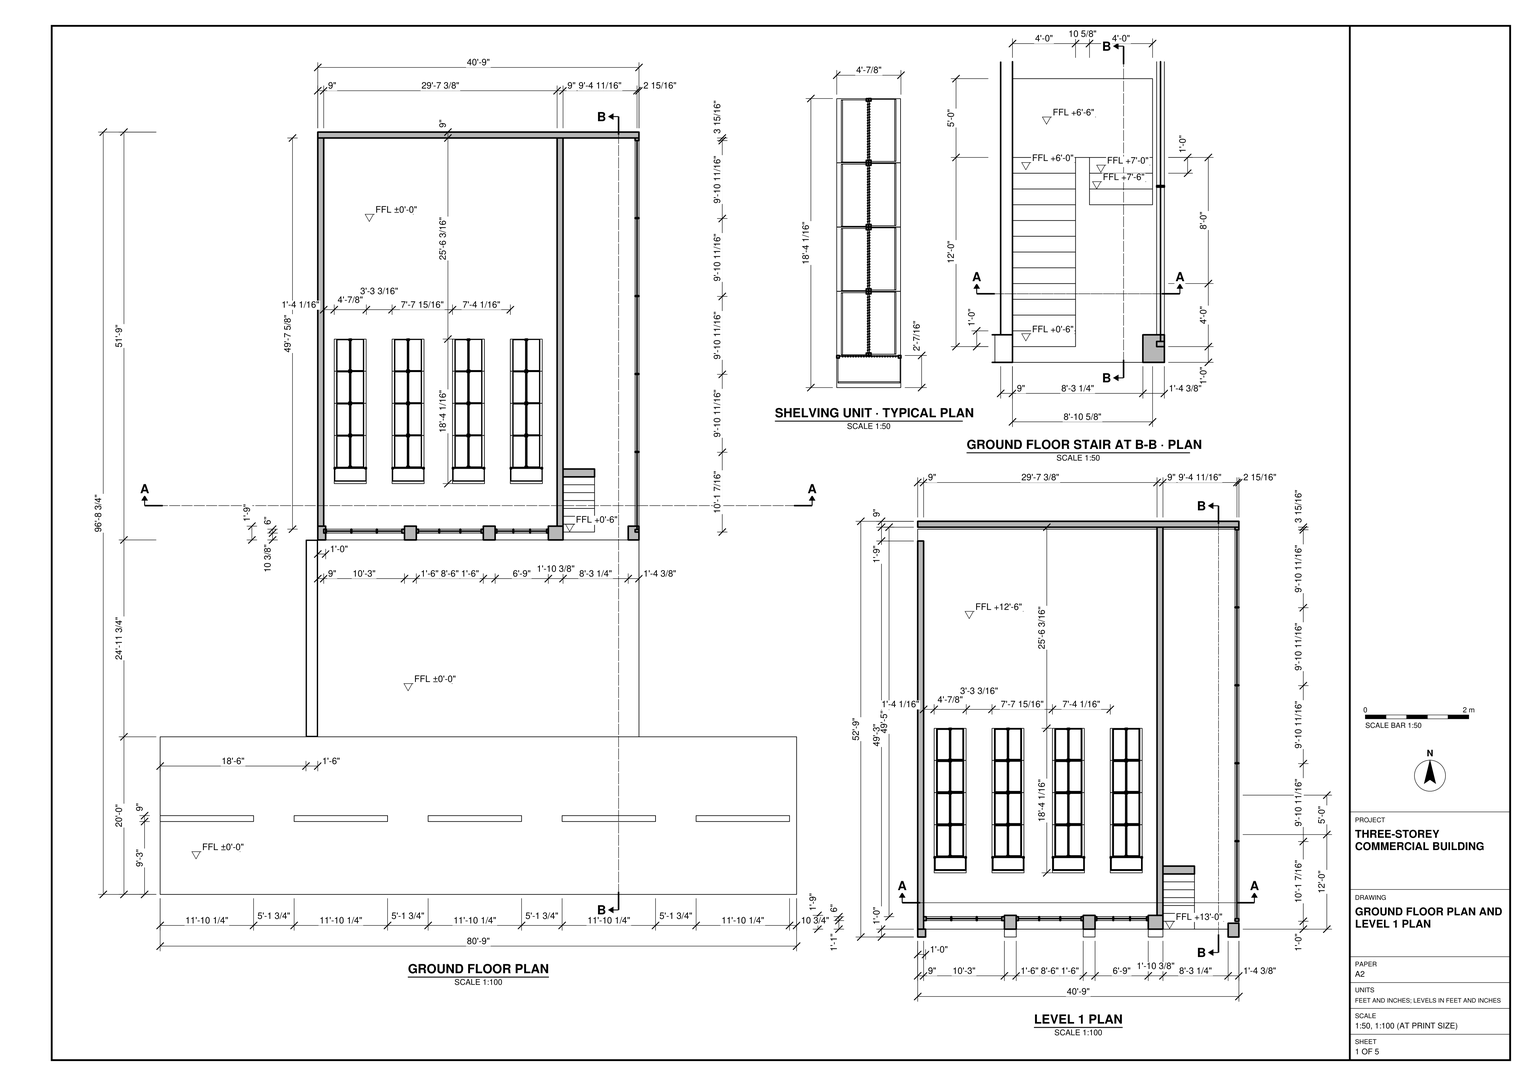
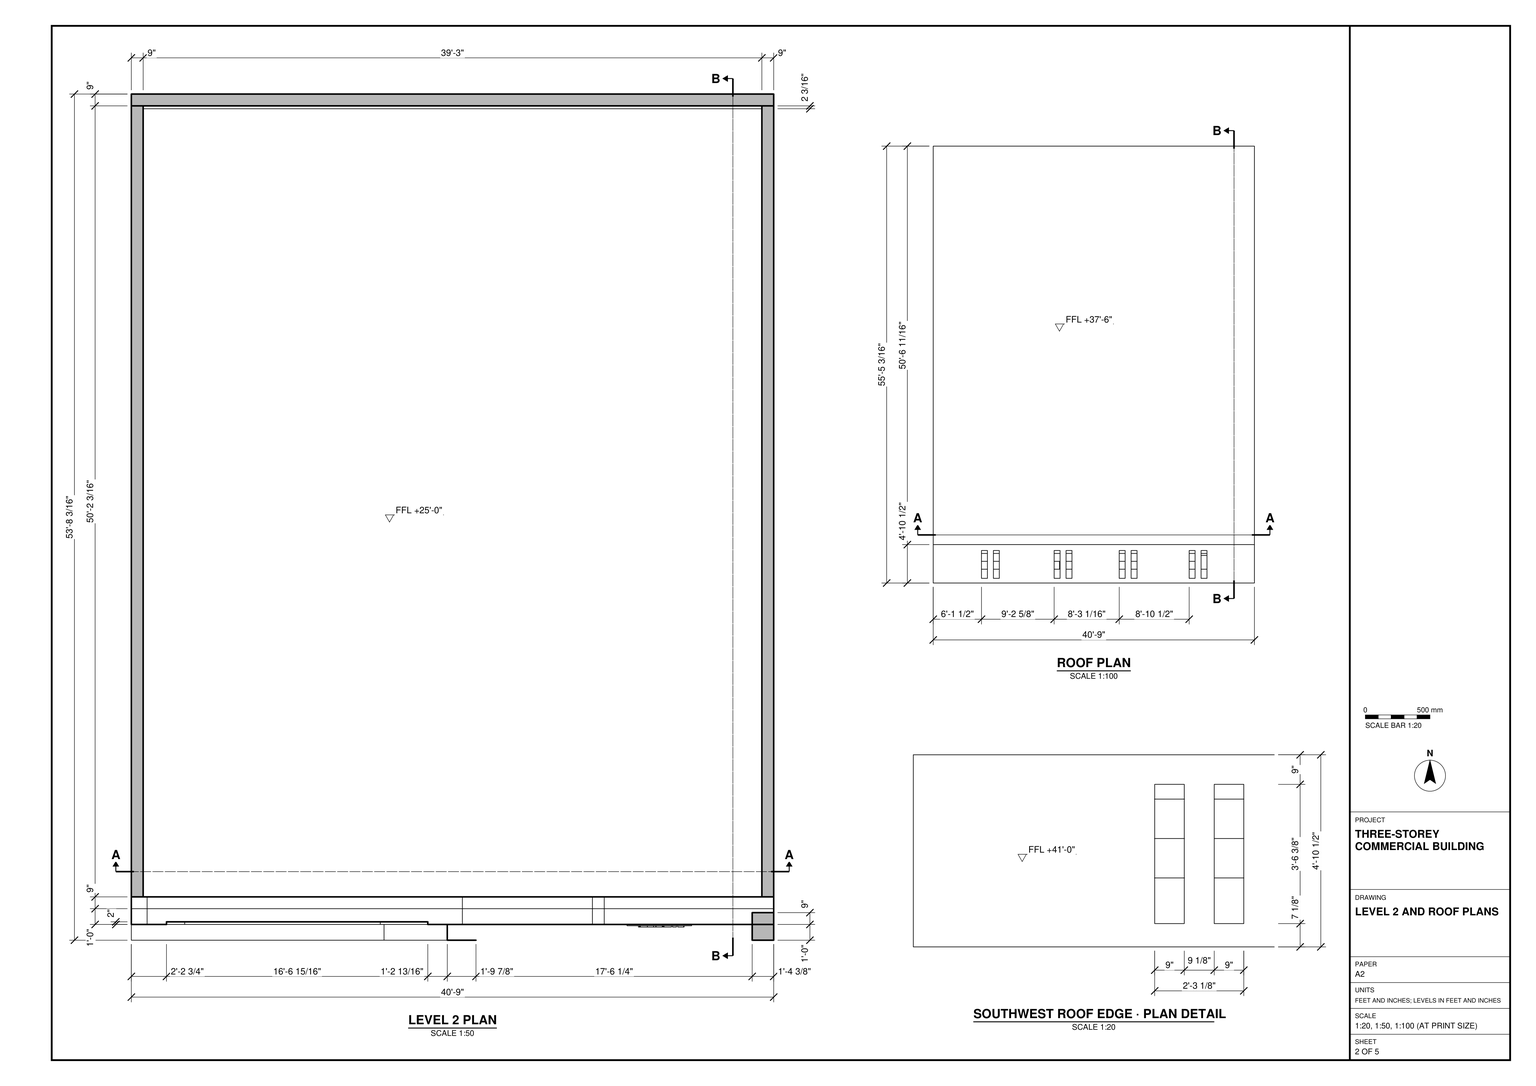
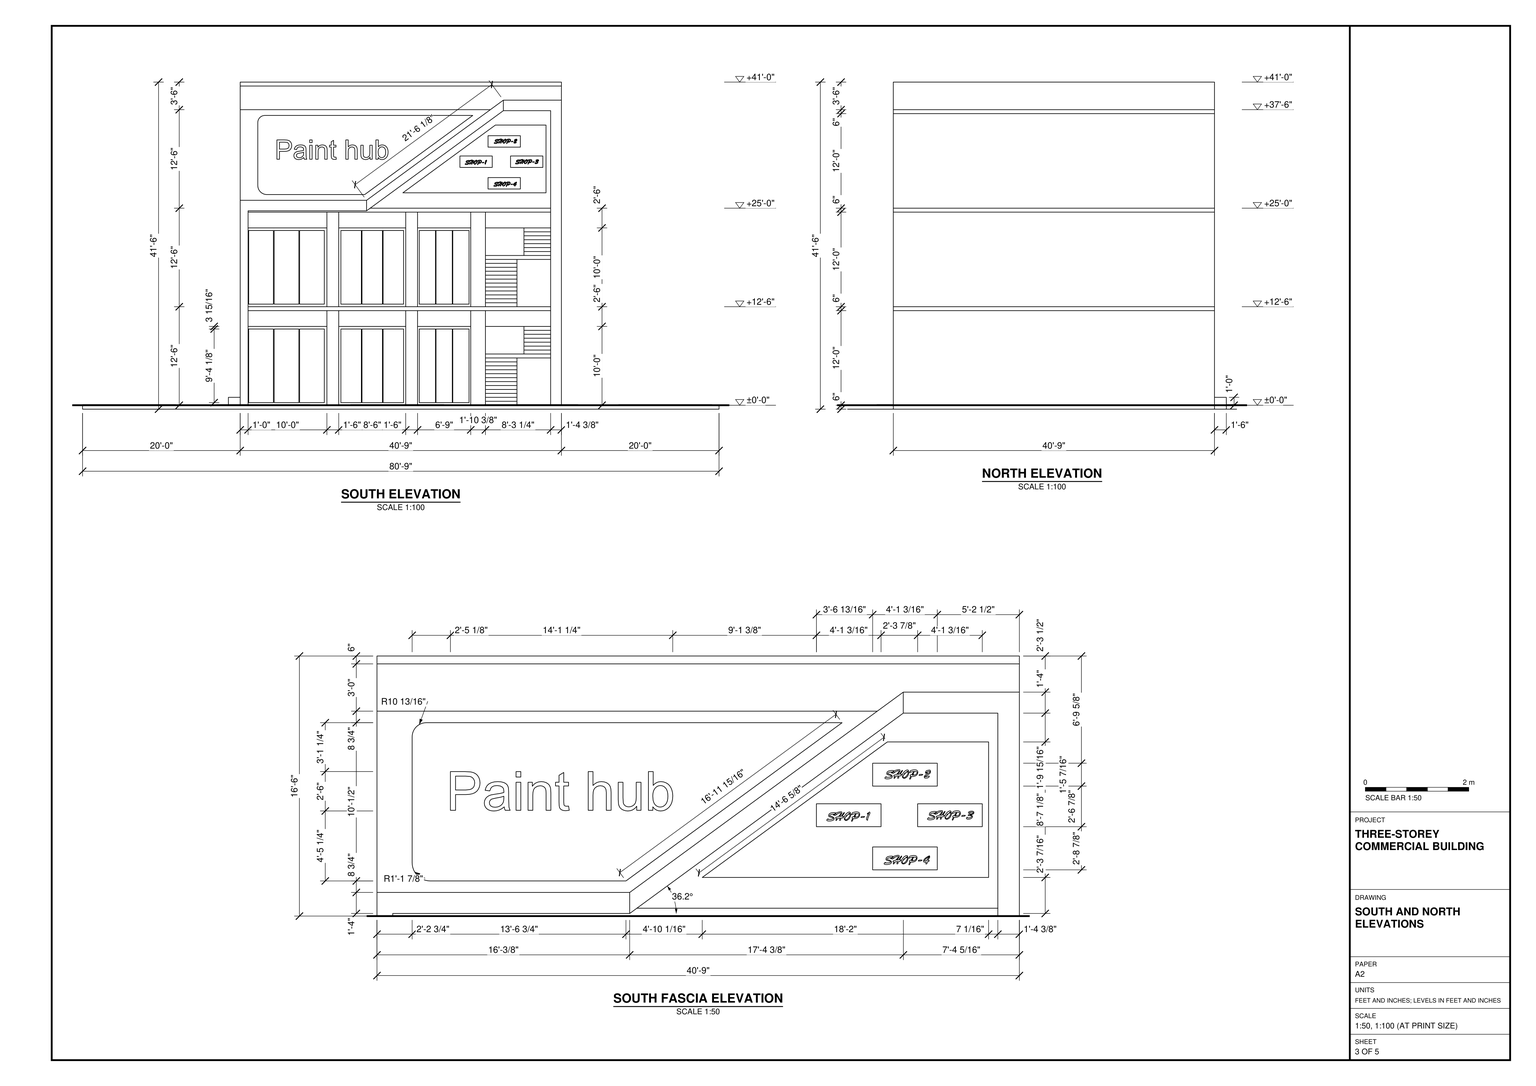
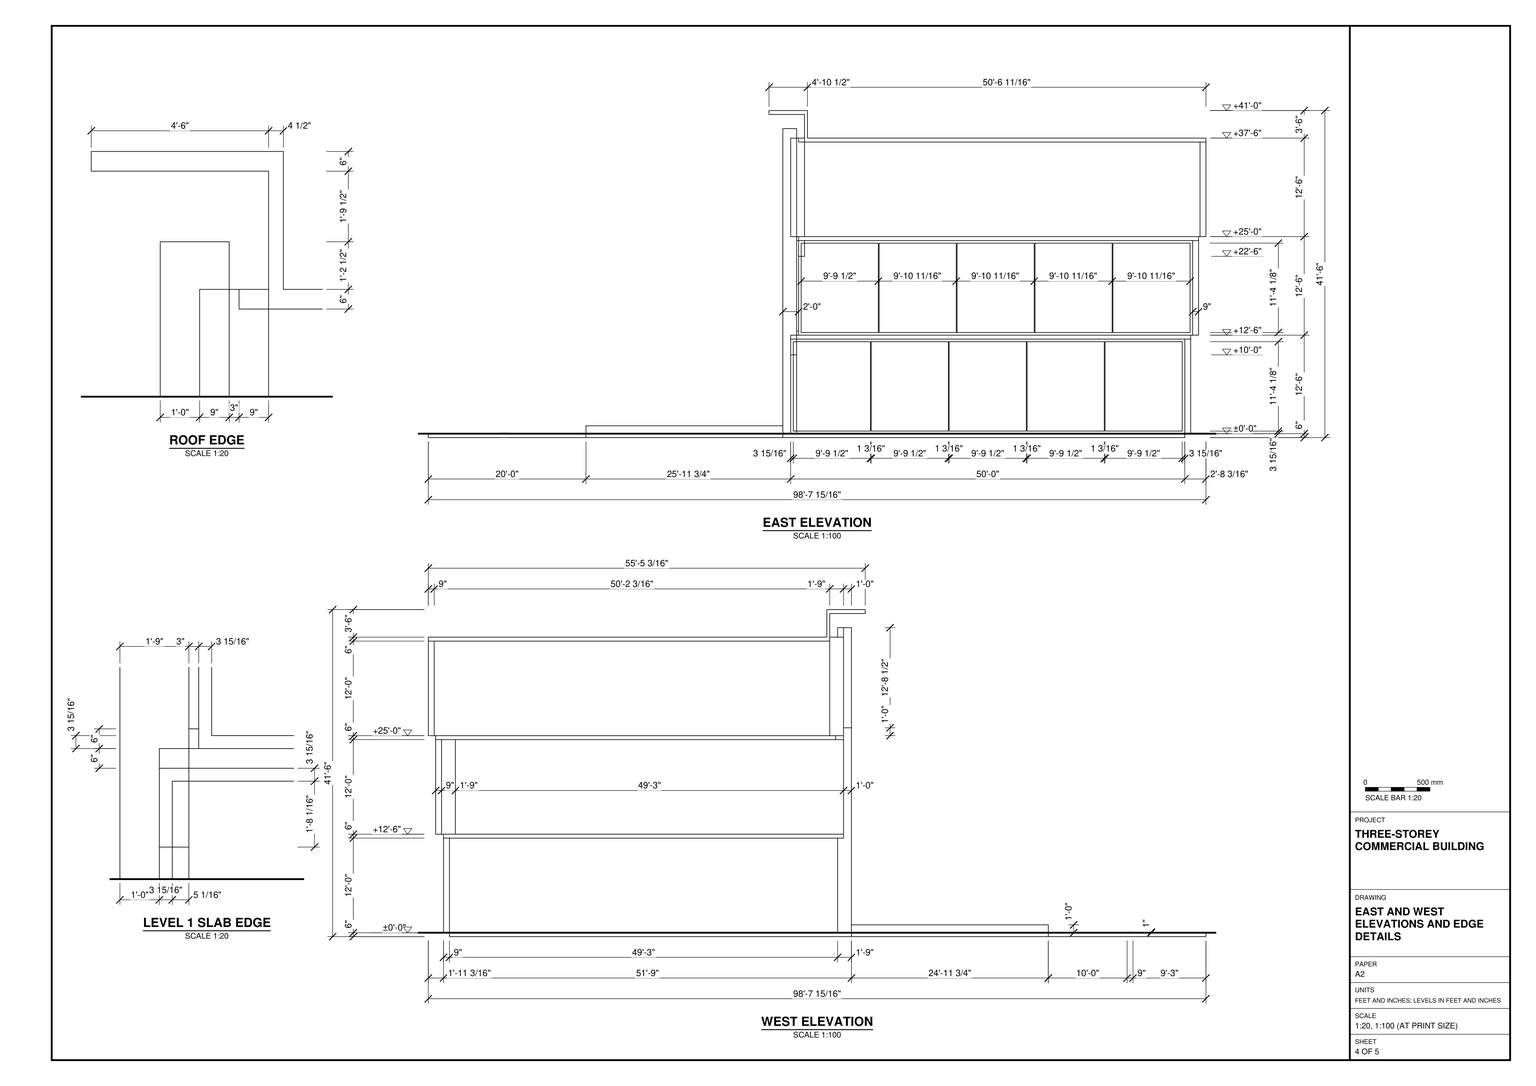
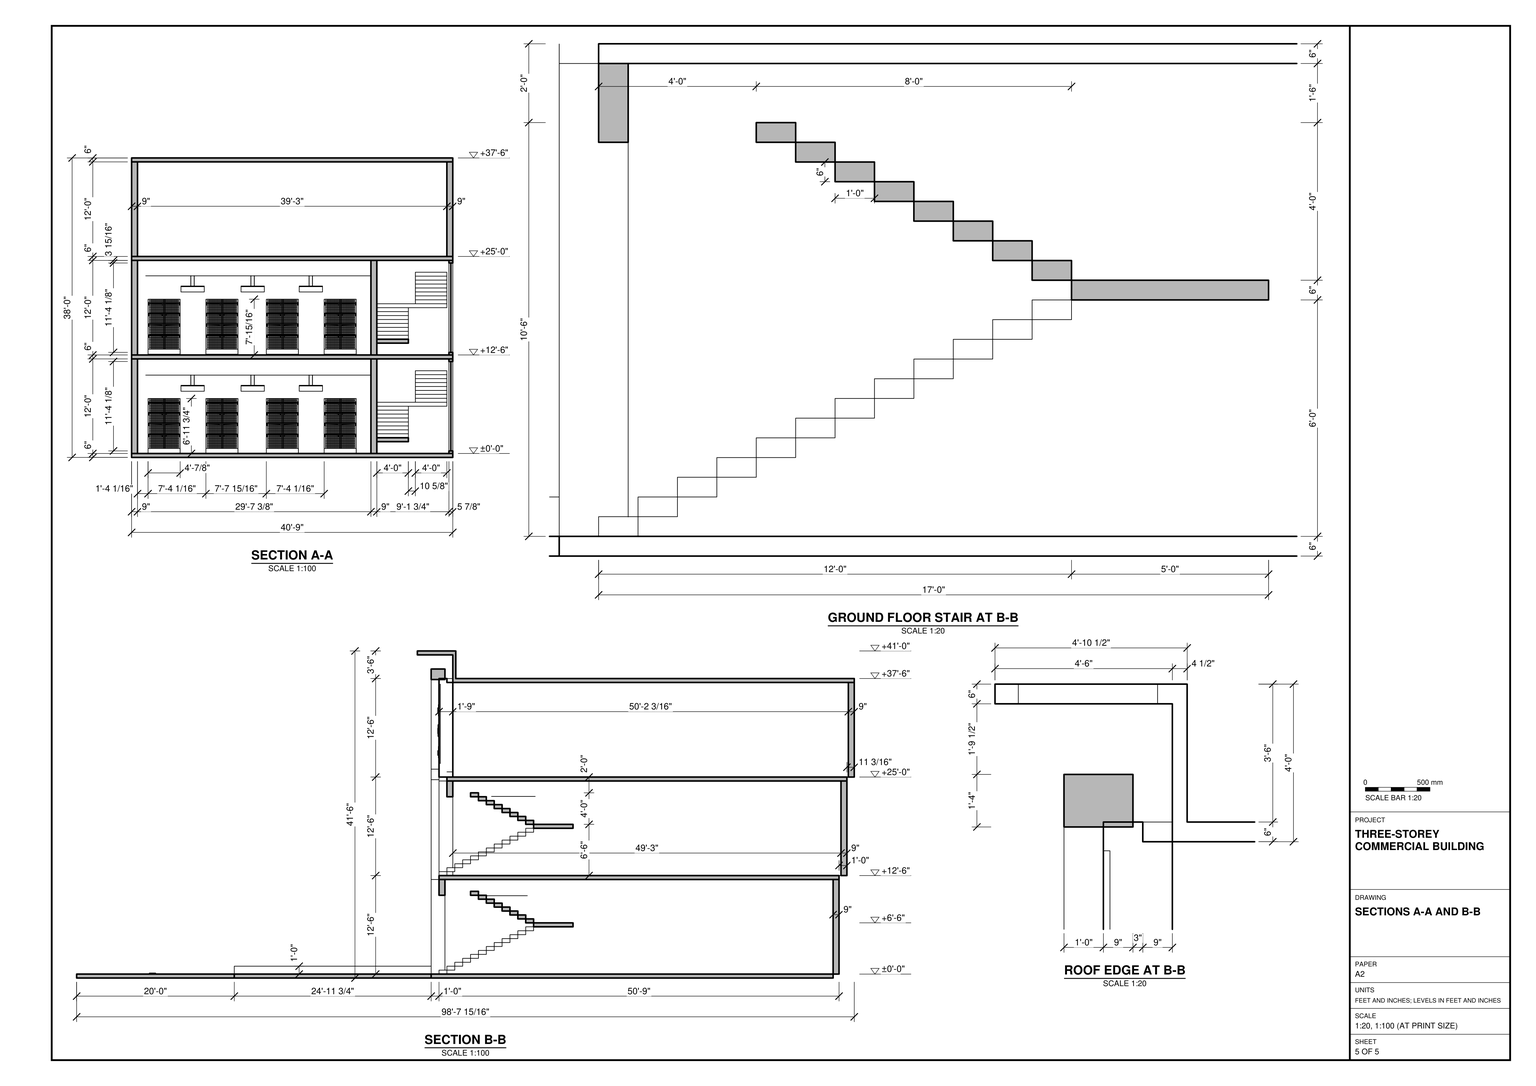
Build the three-storey commercial building and its forecourt in SketchUp using task_files/diagram_01.pdf. Work in feet and inches. Including the forecourt and base, the model measures 80'-9" across the frontage, 98'-7 15/16" from front to back and 41'-6" in total height. Set the storey levels at ±0'-0", +12'-6" and +25'-0". Use +37'-6" for the flat roof level; the raised front roof edge is at +41'-0".

Center the 40'-9" building frontage behind the wide forecourt and include the five narrow strips shown across its front portion. Model the floor slabs, columns, walls at their drawn thicknesses, and door and window openings. On the two lower storeys, form the three glazed shopfront bays facing south, with the stair bay to their right. Use the stair detail to lay out the returning flights, treads and landings. Place four parallel display shelving units on each of the two lower sales floors, matching the typical shelving plan. Leave the level at +25'-0" open inside as drawn.

Use the south fascia elevation to shape the large sign panel, its diagonal division and the four smaller sign panels. Follow the roof plan for the paired details along the front edge. Keep shell elements such as walls, slabs and roof, and each furniture or joinery piece, in separate groups or components; use components for repeated parts. Any decor or loose items shown may be represented by suitable library components. Save one SketchUp model as output_files/three_storey_retail_building_with_shopfronts.skp.

# SketchUp Ruby script. Lengths in inches.
U = 1.inch
M = Sketchup.active_model
def pt(a) = Geom::Point3d.new(a.map { |v| v * U })
def face(e, loops, mat)
  f = e.add_face(loops[0].map { |a| pt(a) })
  loops[1..].each { |l| e.add_face(l.map { |a| pt(a) }).erase! }
  f.material = f.back_material = mat if mat
  f
end
# faces: each face lists its corners as indices into pts; further lists are holes
def faces(e, pts, list, mat = nil) = list.each { |f| face(e, (f[0].is_a?(Array) ? f : [f]).map { |l| l.map { |i| pts[i] } }, mat) }
# xy, xz, yz: faces in a plane at the given z, y or x. An outline is a flat list of corners, or four numbers for a rectangle; further outlines are holes
def ring(l) = l.size == 4 ? [[l[0], l[1]], [l[2], l[1]], [l[2], l[3]], [l[0], l[3]]] : l.each_slice(2).to_a
def flat(e, list, mat, &to3) = list.each { |f| face(e, (f[0].is_a?(Array) ? f : [f]).map { |l| ring(l).map { |u, v| to3.(u, v) } }, mat) }
def xy(e, z, list, mat = nil) = flat(e, list, mat) { |x, y| [x, y, z] }
def xz(e, y, list, mat = nil) = flat(e, list, mat) { |x, z| [x, y, z] }
def yz(e, x, list, mat = nil) = flat(e, list, mat) { |y, z| [x, y, z] }
def lines(e, pts, list) = list.each { |a, b| e.add_line(pt(pts[a]), pt(pts[b])) }
# prism: a flat outline (further loops are holes) pulled along v
def prism(e, loops, v, mat = nil)
  f = face(e, loops, mat); d = Geom::Vector3d.new(v.map { |x| x * U })
  f.pushpull(f.normal.samedirection?(d) ? d.length : -d.length)
end
def box(e, o, s, mat = nil) = prism(e, [[o, [o[0] + s[0], o[1], o[2]], [o[0] + s[0], o[1] + s[1], o[2]], [o[0], o[1] + s[1], o[2]]]], [0, 0, s[2]], mat)
def at(x, y, z, deg = 0) = Geom::Transformation.translation(pt([x, y, z])) * Geom::Transformation.rotation(ORIGIN, Z_AXIS, deg.degrees)
def axes(o, x, y, z) = Geom::Transformation.new([*x, 0, *y, 0, *z, 0, *pt(o).to_a, 1])
def part(name) = M.definitions.add(name)
# library, detail: a bought-in or finely detailed component or shape, given as its bounding box
def library(name, o, s) = part(name).tap { |d| box(d.entities, o, s) }
def detail(e, o, s) = box(e.add_group.entities, o, s)
def put(e, d, t, mat = nil) = e.add_instance(d, t).tap { |i| i.material = mat if mat }
def group(e, t, mat = nil) = e.add_group.tap { |g| g.transformation = t; g.material = mat if mat }.entities
root = M.entities
M.materials.add("[Color A02]").color = [255, 153, 153]
M.materials.add("[Color C05]").color = [255, 127, 0]
M.materials.add("[Color M06]").color = [86, 86, 86]
M.materials.add("[Color M08]").color = [30, 30, 30]
M.materials.add("[Metal_Corrogated_Shiny]").color = [193, 193, 193]
M.materials.add("[Stone Masonry Multi]").color = [182, 175, 164]
M.materials.add("[Translucent Glass Gray]").color = [128, 128, 128]
M.materials["[Translucent Glass Gray]"].alpha = 0.5
M.materials.add("[Translucent_Glass_Tinted]").color = [8, 201, 241]
M.materials["[Translucent_Glass_Tinted]"].alpha = 0.24
c1 = library("Paint hub\#1",[3.18,0,0],[169.25,29.98,1])
c2 = library("Single-sided shelving run",[0,0,0],[24.45,195.63,83.73])
c3 = library("Library component",[0,0,0],[48.9,24.45,83.73])
c4 = part("Double-sided gondola shelving")
put(c4.entities,c2,at(24.45,219.96,0,-180))
put(c4.entities,c2,at(24.13,24.45,0))
put(c4.entities,c3,at(0,0,0))
c5 = part("Sign support rod")
xy(c5.entities,0,[[0.07,0,0.05,0.01,0.01,0.05,0,0.07,0,0.125,0.01,0.15,0.03,0.17,0.07,0.19,0.1,0.2,0.15,0.18,0.17,0.17,0.18,0.15,0.2,0.1,0.19,0.07,0.17,0.03,0.15,0.01,0.125,0]])
xy(c5.entities,15.75,[[0.07,0,0.125,0,0.15,0.01,0.17,0.03,0.19,0.07,0.2,0.1,0.18,0.15,0.17,0.17,0.15,0.18,0.1,0.2,0.07,0.19,0.03,0.17,0.01,0.15,0,0.125,0,0.07,0.01,0.05,0.05,0.01]])
xz(c5.entities,0,[[0.07,0,0.1,15.75],[0.1,0,0.125,15.75]],"[Metal_Corrogated_Shiny]")
yz(c5.entities,0,[[0.07,0,0.1,15.75],[0.1,0,0.125,15.75]],"[Metal_Corrogated_Shiny]")
p = [[0.01,0.05,0],[0.03,0.03,0],[0.03,0.03,15.75],[0.01,0.05,15.75],[0.05,0.01,0],[0.05,0.01,15.75],
  [0.07,0,0],[0.07,0,15.75],[0,0.07,0],[0,0.07,15.75],[0.15,0.01,0],[0.17,0.03,0],
  [0.17,0.03,15.75],[0.15,0.01,15.75],[0.125,0,0],[0.125,0,15.75],[0.18,0.05,0],[0.18,0.05,15.75],
  [0.19,0.07,0],[0.19,0.07,15.75],[0.03,0.17,0],[0.01,0.15,0],[0.01,0.15,15.75],[0.03,0.17,15.75],
  [0,0.125,0],[0,0.125,15.75],[0.2,0.1,0],[0.19,0.125,0],[0.19,0.125,15.75],[0.2,0.1,15.75],
  [0.18,0.15,0],[0.18,0.15,15.75],[0.17,0.17,0],[0.17,0.17,15.75],[0.07,0.19,0],[0.05,0.18,0],
  [0.05,0.18,15.75],[0.07,0.19,15.75],[0.1,0.2,0],[0.1,0.2,15.75],[0.125,0.19,0],[0.125,0.19,15.75],
  [0.15,0.18,0],[0.15,0.18,15.75]]
faces(c5.entities,p,[[0,1,2,3],[1,4,5,2],[4,6,7,5],[8,0,3,9],[10,11,12,13],[14,10,13,15],[11,16,17,12],[16,18,19,17],
  [20,21,22,23],[21,24,25,22],[26,27,28,29],[27,30,31,28],[18,26,29,19],[30,32,33,31],[34,35,36,37],[35,20,23,36],
  [38,34,37,39],[40,38,39,41],[42,40,41,43],[32,42,43,33]],"[Metal_Corrogated_Shiny]")
c6 = part("Paired sign supports")
put(c6.entities,c5,at(5.14,0,0),"[Metal_Corrogated_Shiny]")
put(c6.entities,c5,at(0,0,0),"[Metal_Corrogated_Shiny]")
c7 = part("Uung_P_signage")
xy(c7.entities,0,[[0,0,35.43,0.16]])
xy(c7.entities,8.07,[[0,-0.04,35.43,0],[0,0.16,35.43,0.2]])
xy(c7.entities,9.06,[[0,-0.04,35.43,0.2]])
xz(c7.entities,-0.04,[[0,8.07,35.43,9.06]],"[Metal_Corrogated_Shiny]")
xz(c7.entities,0.16,[[0,0,35.43,8.07]])
xz(c7.entities,0.2,[[0,8.07,35.43,9.06]],"[Metal_Corrogated_Shiny]")
yz(c7.entities,0,[[0,0,0,8.07,-0.04,8.07,-0.04,9.06,0.2,9.06,0.2,8.07,0.16,8.07,0.16,0]])
yz(c7.entities,35.43,[[0,0,0.16,0,0.16,8.07,0.2,8.07,0.2,9.06,-0.04,9.06,-0.04,8.07,0,8.07]])
p = [[-0.07,0,8.07],[0,0,8.07]]
lines(c7.entities,p,[[0,1]])
put(c7.entities,c6,at(14.91,0.125,9.06),"[Metal_Corrogated_Shiny]")
c8 = part("Uung_P_signage\#2")
xy(c8.entities,0,[[0,0,35.43,0.16]])
xy(c8.entities,8.07,[[0,-0.04,35.43,0],[0,0.16,35.43,0.2]])
xy(c8.entities,9.06,[[0,-0.04,35.43,0.2]])
xz(c8.entities,-0.04,[[0,8.07,35.43,9.06]],"[Metal_Corrogated_Shiny]")
xz(c8.entities,0.16,[[0,0,35.43,8.07]])
xz(c8.entities,0.2,[[0,8.07,35.43,9.06]],"[Metal_Corrogated_Shiny]")
yz(c8.entities,0,[[0,0,0,8.07,-0.04,8.07,-0.04,9.06,0.2,9.06,0.2,8.07,0.16,8.07,0.16,0]])
yz(c8.entities,35.43,[[0,0,0.16,0,0.16,8.07,0.2,8.07,0.2,9.06,-0.04,9.06,-0.04,8.07,0,8.07]])
p = [[-0.07,0,8.07],[0,0,8.07]]
lines(c8.entities,p,[[0,1]])
put(c8.entities,c6,at(14.91,0.125,9.06),"[Metal_Corrogated_Shiny]")
c9 = part("Uung_P_signage\#1")
xy(c9.entities,0,[[0,0,35.43,0.16]])
xy(c9.entities,8.07,[[0,-0.04,35.43,0],[0,0.16,35.43,0.2]])
xy(c9.entities,9.06,[[0,-0.04,35.43,0.2]])
xz(c9.entities,-0.04,[[0,8.07,35.43,9.06]],"[Metal_Corrogated_Shiny]")
xz(c9.entities,0.2,[[0,8.07,35.43,9.06]],"[Metal_Corrogated_Shiny]")
yz(c9.entities,0,[[0,0,0,8.07,-0.04,8.07,-0.04,9.06,0.2,9.06,0.2,8.07,0.16,8.07,0.16,0]])
yz(c9.entities,35.43,[[0,0,0.16,0,0.16,8.07,0.2,8.07,0.2,9.06,-0.04,9.06,-0.04,8.07,0,8.07]])
p = [[-0.07,0,8.07],[0,0,8.07]]
lines(c9.entities,p,[[0,1]])
put(c9.entities,c6,at(14.91,0.125,9.06),"[Metal_Corrogated_Shiny]")
c10 = part("Component\#14")
xy(c10.entities,0,[[0,0,403.78,66.61]])
c11 = part("FIXTURE+GONDOLA+SET_DO")
put(c11.entities,c4,at(-0.98,-23.62,-0.06))
put(c11.entities,c4,at(87.09,-23.62,-0.06))
put(c11.entities,c7,at(49.14,0,94.66))
put(c11.entities,c8,at(-130.9,0,94.66))
put(c11.entities,c4,at(-92.95,-23.62,-0.06))
put(c11.entities,c4,at(-181.02,-23.62,-0.06))
put(c11.entities,c9,at(-39.45,0,94.66))
put(c11.entities,c10,axes([-184.625,-29.51,119.25],[0.87,0,0],[0,1,0],[0,0,1]),"[Translucent_Glass_Tinted]")
c12 = library("SHOP-2",[0.1,0,0],[34.76,7.3125,1])
c13 = library("SHOP-3",[0.1,0,0],[35.35,7.3125,1])
c14 = library("SHOP-4",[0.1,0,0],[34.74,7.3125,1])
c15 = library("SHOP-1",[0.1,0,0],[32.9,7.3125,1])
c16 = part("Group\#14")
box(c16.entities,[-231,0,0],[591,9,144])
c17 = part("Group\#3")
box(c17.entities,[-9,0,0],[489,9,144])
c18 = part("Group\#16")
box(c18.entities,[0,0,0],[9,591,144])
c19 = part("Group\#19")
box(c19.entities,[0,0,0],[48,12,6])
c20 = part("Group\#18")
put(c20.entities,c19,at(0,24,12))
put(c20.entities,c19,at(0,0,0))
put(c20.entities,c19,at(0,12,6))
put(c20.entities,c19,at(0,36,18))
put(c20.entities,c19,at(0,48,24))
put(c20.entities,c19,at(0,60,30))
put(c20.entities,c19,at(0,72,36))
put(c20.entities,c19,at(0,84,42))
put(c20.entities,c19,at(0,96,48))
put(c20.entities,c19,at(0,108,54))
put(c20.entities,c19,at(0,120,60))
put(c20.entities,c19,at(0,132,66))
g1 = group(c20.entities,at(0,144,72))
box(g1,[0,0,0],[106.625,60,6])
put(c20.entities,c19,at(58.625,132,78))
put(c20.entities,c19,at(58.625,120,84))
put(c20.entities,c19,at(58.625,108,90))
put(c20.entities,c19,at(58.625,96,96))
put(c20.entities,c19,at(58.625,84,102))
put(c20.entities,c19,at(58.625,72,108))
put(c20.entities,c19,at(58.625,60,114))
put(c20.entities,c19,at(58.625,48,120))
c21 = part("Group25\#2")
xy(c21.entities,0,[[-57.5625,-56.0625,-19.98,56.0625],[-18.79,-56.0625,18.79,56.0625],[19.98,-56.0625,57.5625,56.0625]])
c22 = part("Group24\#1")
prism(c22.entities,[[[61.5,-60,0],[-61.5,-60,0],[-61.5,60,0],[61.5,60,0]],[[19.98,-56.0625,0],[57.5625,-56.0625,0],[57.5625,56.0625,0],[19.98,56.0625,0]],[[18.79,56.0625,0],[-18.79,56.0625,0],[-18.79,-56.0625,0],[18.79,-56.0625,0]],[[-19.98,-56.0625,0],[-19.98,56.0625,0],[-57.5625,56.0625,0],[-57.5625,-56.0625,0]]],[0,0,5.875])
put(c22.entities,c21,at(0,0,2.9375),"[Translucent Glass Gray]")
c23 = part("Group\#20")
p = [[0,0,120],[0,0.1,0],[123,0.1,0],[123,0,120]]
lines(c23.entities,p,[[0,1],[1,2],[2,3],[3,0]])
put(c23.entities,c22,axes([61.5,5.93,60.01],[1,0,0],[0,-0.00086,1],[0,-1,-0.00086]),"[Color M06]")
c24 = part("Group\#21")
put(c24.entities,c23,at(0,0,0))
put(c24.entities,c23,axes([141,0,0],[0.82927,0,0],[0,1,0],[0,0,1]))
put(c24.entities,c23,axes([261,0,0],[0.65854,0,0],[0,1,0],[0,0,1]))
c25 = part("Group57\#2")
xy(c25.entities,0,[[-296.0625,-68.0625,-178.59,68.0625],[-177.4,-68.0625,-59.92,68.0625],[-58.74,-68.0625,58.74,68.0625],[59.93,-68.0625,177.4,68.0625],[178.59,-68.0625,296.0625,68.0625]])
c26 = part("Group56\#1")
prism(c26.entities,[[[300,72,0],[300,-72,0],[-300,-72,0],[-300,72,0]],[[59.93,68.0625,0],[59.93,-68.0625,0],[177.4,-68.0625,0],[177.4,68.0625,0]],[[58.74,68.0625,0],[-58.74,68.0625,0],[-58.74,-68.0625,0],[58.74,-68.0625,0]],[[-59.92,-68.0625,0],[-59.92,68.0625,0],[-177.4,68.0625,0],[-177.4,-68.0625,0]],[[178.59,68.0625,0],[178.59,-68.0625,0],[296.0625,-68.0625,0],[296.0625,68.0625,0]],[[-296.0625,-68.0625,0],[-178.59,-68.0625,0],[-178.59,68.0625,0],[-296.0625,68.0625,0]]],[0,0,5.875])
put(c26.entities,c25,at(0,0,2.9375),"[Translucent Glass Gray]")
c27 = part("Group\#1")
put(c27.entities,c26,axes([60,3.125,72],[-1,0,0],[0,0,1],[0,1,0]))
c28 = part("Group\#23")
box(c28.entities,[0,0,0],[142.23,9,1])
c29 = part("Group\#24")
box(c29.entities,[0,0,0],[49.1875,1,17.4375])
put(root,c1,axes([292.72,553.75,374.03],[1,0,0],[0,0,1],[0,-1,0]))
put(root,c11,at(446.07,649.14,0.08))
put(root,c11,at(446.07,661.14,151.27))
put(root,c12,axes([626.53,550.75,398.19],[1,0,0],[0,0,1],[0,-1,0]))
put(root,c13,axes([658.95,550.75,367.01],[1,0,0],[0,0,1],[0,-1,0]))
put(root,c14,axes([625.94,550.75,332.98],[1,0,0],[0,0,1],[0,-1,0]))
put(root,c15,axes([582.29,550.75,366.125],[1,0,0],[0,0,1],[0,-1,0]))
g2 = group(root,at(240,539.75,-6))
g3 = group(g2,at(0,12,6),"[Color C05]")
xy(g3,0,[[0,-12,12,9],[132,-12,150,9],[252,-12,270,9],[351,-12,360,9],[360,-12,373.375,9],
  [472.625,-12,475.625,9],[475.625,-12,489,9]])
xy(g3,120,[[12,0,132,9],[150,0,252,9],[270,0,351,9],[373.375,0,489,5.0625],[373.375,5.0625,489,9]])
xy(g3,144,[[132,-12,150,0],[252,-12,270,0],[351,-12,373.375,0],[0,0,360,9],[360,0,472.625,9],
  [472.625,0,489,9]])
xy(g3,296,[[12,-12,192.375,0]])
xy(g3,312,[[0,-12,192.375,0]])
xy(g3,448.5,[[400.625,-12,472.625,9]])
xy(g3,464.5,[[400.625,-12,489,9]],"[Color C05]")
xz(g3,-12,[[132,0,150,144],[252,0,270,144],[351,0,373.375,144]])
xz(g3,-12,[[0,0,12,0,12,296,192.375,296,192.375,312,0,312],[472.625,0,489,0,489,464.5,400.625,464.5,400.625,448.5,472.625,448.5],[192.375,296,400.625,448.5,400.625,464.5,192.375,312]],"[Color C05]")
xz(g3,0,[[12,120,132,144],[150,120,252,144],[270,120,351,144],[373.375,120,489,144],[0,144,0,312,192.375,312,192.375,296,12,296,12,144]])
xz(g3,9,[[0,0,0,144,472.625,144,472.625,120,373.375,120,373.375,0,351,0,351,120,270,120,270,0,252,0,252,120,150,120,150,0,132,0,132,120,12,120,12,0],[472.625,0,489,120],[472.625,120,489,144],[472.625,144,472.625,448.5,400.625,448.5,400.625,464.5,489,464.5,489,144]])
yz(g3,0,[[-12,0,-12,312,0,312,0,144,9,144,9,0]],"[Color C05]")
yz(g3,12,[[-12,0,9,0,9,120,0,120,0,296,-12,296]])
yz(g3,132,[[-12,0,-12,144,0,144,0,120,9,120,9,0]])
yz(g3,150,[[-12,0,9,0,9,120,0,120,0,144,-12,144]])
yz(g3,192.375,[[-12,296,0,312]])
yz(g3,252,[[-12,0,-12,144,0,144,0,120,9,120,9,0]])
yz(g3,270,[[-12,0,9,0,9,120,0,120,0,144,-12,144]])
yz(g3,351,[[-12,0,-12,144,0,144,0,120,9,120,9,0]])
yz(g3,373.375,[[-12,0,9,0,9,120,0,120,0,144,-12,144]])
yz(g3,400.625,[[-12,448.5,9,464.5]],"[Color C05]")
yz(g3,472.625,[[-12,0,9,448.5]],"[Color C05]")
yz(g3,489,[[-12,0,9,0,9,120,0,120,0,144,9,144,9,464.5,-12,464.5],[0,120,9,144]])
p = [[400.625,-12,464.5],[400.625,0,464.5],[192.375,0,312],[192.375,-12,312]]
faces(g3,p,[[0,1,2,3]],"[Color C05]")
put(g2,c16,at(0,381,6,-90))
put(g2,c17,at(9,612,6))
g4 = group(g2,at(0,12,150))
box(g4,[0,0,0],[489,609,6])
g5 = group(g2,at(0,0,0))
box(g5,[0,0,0],[489,612,6])
g6 = group(root,at(240,562.9375,294))
g7 = group(g6,at(480,372,6,-90))
box(g7,[-240,0,0],[602.1875,9,144])
g8 = group(g6,at(0,381,6,-90))
box(g8,[-231,0,0],[602.1875,9,144])
put(g6,c17,at(9,612,6))
g9 = group(g6,at(0,12,150))
xy(g9,0,[[0,-2.1875,489,609]])
xy(g9,6,[[0,2.3125,489,609]])
xy(g9,42,[[[0,-56.1875,489,-2.1875],[73.5,-49.09,82.5,-6.6875],[91.625,-49.09,100.625,-6.6875],[184.125,-49.09,193.125,-6.6875],[202.25,-49.09,211.25,-6.6875],[301.3125,-49.09,310.3125,-6.6875],[283.1875,-49.09,292.1875,-6.6875],[389.6875,-49.09,398.6875,-6.6875],[407.8125,-49.09,416.8125,-6.6875]]])
xy(g9,48,[[[0,-56.1875,489,2.3125],[73.5,-49.09,82.5,-6.6875],[91.625,-49.09,100.625,-6.6875],[202.25,-49.09,211.25,-6.6875],[184.125,-49.09,193.125,-6.6875],[301.3125,-49.09,310.3125,-6.6875],[283.1875,-49.09,292.1875,-6.6875],[407.8125,-49.09,416.8125,-6.6875],[389.6875,-49.09,398.6875,-6.6875]]])
xz(g9,-56.1875,[[0,42,489,48]])
xz(g9,-49.09,[[73.5,42,82.5,48],[91.625,42,100.625,48],[184.125,42,193.125,48],[202.25,42,211.25,48],[283.1875,42,292.1875,48],
  [301.3125,42,310.3125,48],[389.6875,42,398.6875,48],[407.8125,42,416.8125,48]])
xz(g9,-6.6875,[[73.5,42,82.5,48],[91.625,42,100.625,48],[184.125,42,193.125,48],[202.25,42,211.25,48],[283.1875,42,292.1875,48],
  [301.3125,42,310.3125,48],[389.6875,42,398.6875,48],[407.8125,42,416.8125,48]])
xz(g9,-2.1875,[[0,0,489,42]])
xz(g9,2.3125,[[0,6,489,48]])
xz(g9,609,[[0,0,489,6]])
yz(g9,0,[[-2.1875,0,-2.1875,42,-56.1875,42,-56.1875,48,2.3125,48,2.3125,6,609,6,609,0]])
yz(g9,73.5,[[-49.09,42,-6.6875,48]])
yz(g9,82.5,[[-49.09,42,-6.6875,48]])
yz(g9,91.625,[[-49.09,42,-6.6875,48]])
yz(g9,100.625,[[-49.09,42,-6.6875,48]])
yz(g9,184.125,[[-49.09,42,-6.6875,48]])
yz(g9,193.125,[[-49.09,42,-6.6875,48]])
yz(g9,202.25,[[-49.09,42,-6.6875,48]])
yz(g9,211.25,[[-49.09,42,-6.6875,48]])
yz(g9,283.1875,[[-49.09,42,-6.6875,48]])
yz(g9,292.1875,[[-49.09,42,-6.6875,48]])
yz(g9,301.3125,[[-49.09,42,-6.6875,48]])
yz(g9,310.3125,[[-49.09,42,-6.6875,48]])
yz(g9,389.6875,[[-49.09,42,-6.6875,48]])
yz(g9,398.6875,[[-49.09,42,-6.6875,48]])
yz(g9,407.8125,[[-49.09,42,-6.6875,48]])
yz(g9,416.8125,[[-49.09,42,-6.6875,48]])
yz(g9,489,[[-2.1875,0,609,0,609,6,2.3125,6,2.3125,48,-56.1875,48,-56.1875,42,-2.1875,42]])
g10 = group(g6,at(0,0.8125,6))
xy(g10,0,[[0,-12,12,9],[12,-12,252,9],[252,-12,351,9],[351,-12,360,9],[360,-12,489,9]])
xy(g10,20.76,[[40.64,-12,189.51,-10]])
xy(g10,141.24,[[37.54,-12,354.04,-10]])
xy(g10,144,[[360,0,489,9]])
xy(g10,150,[[0,-12,489,0],[0,0,360,9]])
xz(g10,-12,[[[0,0,489,0,489,150,380.82,150,192.375,12,0,12],[247.61,23.42,388.48,126.58,465.58,126.58,465.58,23.42]],[[0,12,192.375,12,380.82,150,0,150],[40.64,20.76,38.83,20.875,37.05,21.23,35.33,21.8125,33.7,22.62,32.1875,23.625,30.82,24.82,29.625,26.1875,28.62,27.7,27.8125,29.33,27.23,31.05,26.875,32.83,26.76,34.64,26.76,130.46,26.85,131.87,27.125,133.25,27.58,134.59,28.2,135.85,28.99,137.02,29.92,138.08,30.98,139.01,32.15,139.8,33.41,140.42,34.75,140.875,36.13,141.15,37.54,141.24,354.04,141.24,189.51,20.76]]])
xz(g10,-12,[[247.61,23.42,465.58,23.42,465.58,126.58,388.48,126.58]],"[Color M06]")
xz(g10,-10,[[40.64,20.76,189.51,20.76,354.04,141.24,37.54,141.24,36.13,141.15,34.75,140.875,33.41,140.42,32.15,139.8,30.98,139.01,29.92,138.08,28.99,137.02,28.2,135.85,27.58,134.59,27.125,133.25,26.85,131.87,26.76,130.46,26.76,34.64,26.875,32.83,27.23,31.05,27.8125,29.33,28.62,27.7,29.625,26.1875,30.82,24.82,32.1875,23.625,33.7,22.62,35.33,21.8125,37.05,21.23,38.83,20.875]],"[Color M06]")
xz(g10,0,[[360,144,489,150]])
xz(g10,9,[[0,0,0,150,360,150,360,144,489,144,489,0]])
yz(g10,0,[[-12,0,9,150]])
yz(g10,26.76,[[-12,34.64,-10,130.46]])
yz(g10,360,[[0,144,9,150]])
yz(g10,489,[[-12,0,9,0,9,144,0,144,0,150,-12,150]])
p = [[38.83,-12,20.875],[40.64,-12,20.76],[40.64,-10,20.76],[38.83,-10,20.875],[189.51,-12,20.76],[354.04,-12,141.24],
  [354.04,-10,141.24],[189.51,-10,20.76],[37.05,-12,21.23],[37.05,-10,21.23],[35.33,-12,21.8125],[35.33,-10,21.8125],
  [33.7,-12,22.62],[33.7,-10,22.62],[32.1875,-12,23.625],[32.1875,-10,23.625],[30.82,-12,24.82],[30.82,-10,24.82],
  [29.625,-12,26.1875],[29.625,-10,26.1875],[28.62,-12,27.7],[28.62,-10,27.7],[27.8125,-12,29.33],[27.8125,-10,29.33],
  [27.23,-12,31.05],[27.23,-10,31.05],[26.875,-12,32.83],[26.875,-10,32.83],[26.76,-12,34.64],[26.76,-10,34.64],
  [26.85,-12,131.87],[26.76,-12,130.46],[26.76,-10,130.46],[26.85,-10,131.87],[27.125,-12,133.25],[27.125,-10,133.25],
  [27.58,-12,134.59],[27.58,-10,134.59],[28.2,-12,135.85],[28.2,-10,135.85],[28.99,-12,137.02],[28.99,-10,137.02],
  [29.92,-12,138.08],[29.92,-10,138.08],[30.98,-12,139.01],[30.98,-10,139.01],[32.15,-12,139.8],[32.15,-10,139.8],
  [33.41,-12,140.42],[33.41,-10,140.42],[34.75,-12,140.875],[34.75,-10,140.875],[36.13,-12,141.15],[36.13,-10,141.15],
  [37.54,-12,141.24],[37.54,-10,141.24],[360,9,7.875],[360,9,0],[360,0,7.875]]
faces(g10,p,[[0,1,2,3],[4,5,6,7],[8,0,3,9],[10,8,9,11],[12,10,11,13],[14,12,13,15],[16,14,15,17],[18,16,17,19],
  [20,18,19,21],[22,20,21,23],[24,22,23,25],[26,24,25,27],[28,26,27,29],[30,31,32,33],[34,30,33,35],[36,34,35,37],
  [38,36,37,39],[40,38,39,41],[42,40,41,43],[44,42,43,45],[46,44,45,47],[48,46,47,49],[50,48,49,51],[52,50,51,53],
  [54,52,53,55]])
lines(g10,p,[[56,57],[56,58]])
put(root,c18,at(604.375,560.75,0))
put(root,c20,at(613.375,551.75,0))
put(root,c20,at(613.375,551.75,150))
put(root,c24,at(249,564.75,150))
put(root,c24,at(249,550.15,0))
g11 = group(root,at(240,240,-6),"[Stone Masonry Multi]")
xy(g11,0,[[-18,0,489,299.75]])
xy(g11,6,[[0,0,489,299.75],[-17,1,-1,298.75]])
xy(g11,18,[[[-18,0,0,299.75],[-17,1,-1,298.75]]])
xz(g11,0,[[-18,0,489,0,489,6,0,6,0,18,-18,18]])
xz(g11,1,[[-17,6,-1,18]])
xz(g11,298.75,[[-17,6,-1,18]])
xz(g11,299.75,[[-18,0,-18,18,0,18,0,6,489,6,489,0]])
yz(g11,-18,[[0,0,299.75,18]])
yz(g11,-17,[[1,6,298.75,18]])
yz(g11,-1,[[1,6,298.75,18]])
yz(g11,0,[[0,6,299.75,18]])
yz(g11,489,[[0,0,299.75,6]])
put(root,c18,at(604.375,572.75,150))
put(root,c16,at(240,911.75,150,-90))
put(root,c27,at(720,923.75,150,-90),"[Color M06]")
put(root,c17,at(249,1163.75,150))
g12 = group(root,at(240,563.75,294))
prism(g12,[[[0,609,0],[489,609,0],[489,0,0],[12,0,0],[12,-12,0],[0,-12,0]]],[0,0,6])
g13 = group(root,at(240,563.75,150))
xy(g13,0,[[132,-12,150,9],[252,-12,270,9],[351,-12,360,9],[360,-12,373.375,9]])
xy(g13,120,[[12,0,132,9],[150,0,252,9],[270,0,351,9],[373.375,0,489,5.0625],[373.375,5.0625,489,9]])
xy(g13,144,[[132,-12,150,0],[252,-12,270,0],[351,-12,373.375,0],[12,0,360,9],[360,0,489,9]])
xz(g13,-12,[[132,0,150,144],[252,0,270,144],[351,0,373.375,144]])
xz(g13,0,[[12,120,132,144],[150,120,252,144],[270,120,351,144],[373.375,120,489,144],[0,144,12,150]])
xz(g13,9,[[132,0,132,120,12,120,12,144,360,144,360,0,351,0,351,120,270,120,270,0,252,0,252,120,150,120,150,0],[360,0,373.375,0,373.375,120,489,120,489,144,360,144]])
yz(g13,132,[[-12,0,-12,144,0,144,0,120,9,120,9,0]])
yz(g13,150,[[-12,0,9,0,9,120,0,120,0,144,-12,144]])
yz(g13,252,[[-12,0,-12,144,0,144,0,120,9,120,9,0]])
yz(g13,270,[[-12,0,9,0,9,120,0,120,0,144,-12,144]])
yz(g13,351,[[-12,0,-12,144,0,144,0,120,9,120,9,0]])
yz(g13,373.375,[[-12,0,9,0,9,120,0,120,0,144,-12,144]])
yz(g13,489,[[0,120,9,144]])
p = [[360,9,7.875],[360,0,7.875]]
lines(g13,p,[[0,1]])
put(root,c27,at(720,911.75,0,-90),"[Color M06]")
g14 = group(root,at(0,0,-6),"[Color M08]")
box(g14,[0,0,0],[969,240,6])
put(root,c28,at(0,111,0))
put(root,c28,at(204,111,0))
put(root,c28,at(408,111,0))
put(root,c28,at(612,111,0))
put(root,c28,at(816,111,0))
put(root,c29,at(617.33,550.75,392.9375),"[Color A02]")
put(root,c29,at(574.51,550.75,362.0625),"[Color A02]")
put(root,c29,at(651.58,550.75,362.0625),"[Color A02]")
put(root,c29,at(617.33,550.75,329.1875),"[Color A02]")
